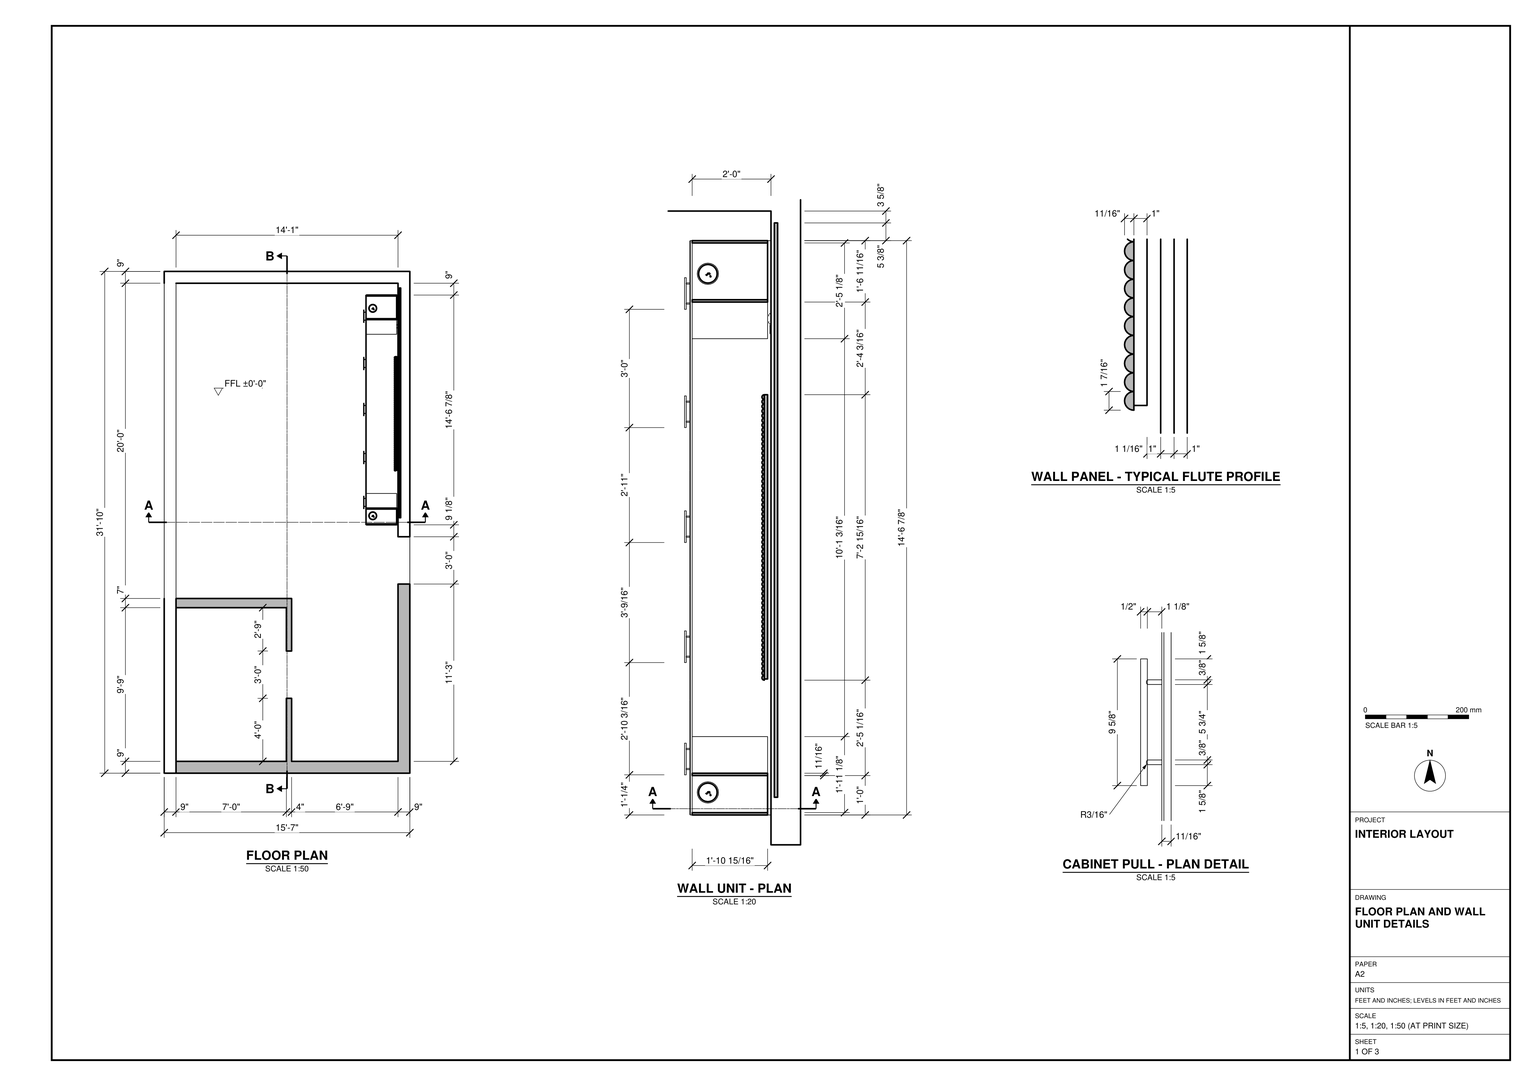
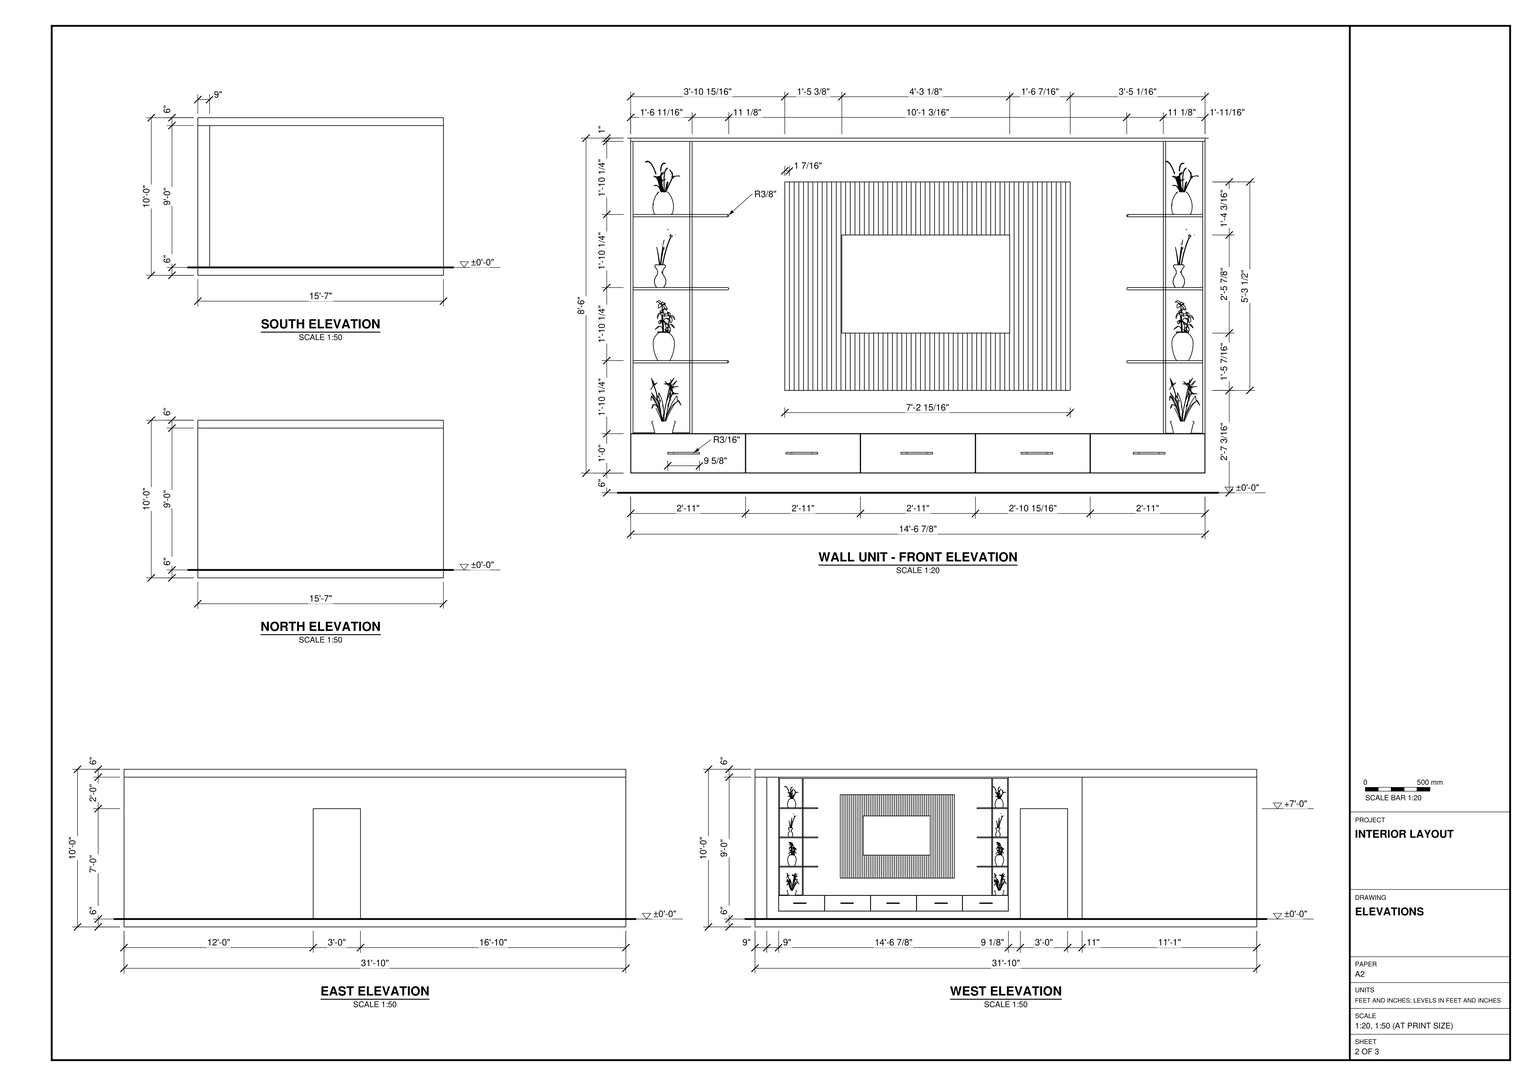
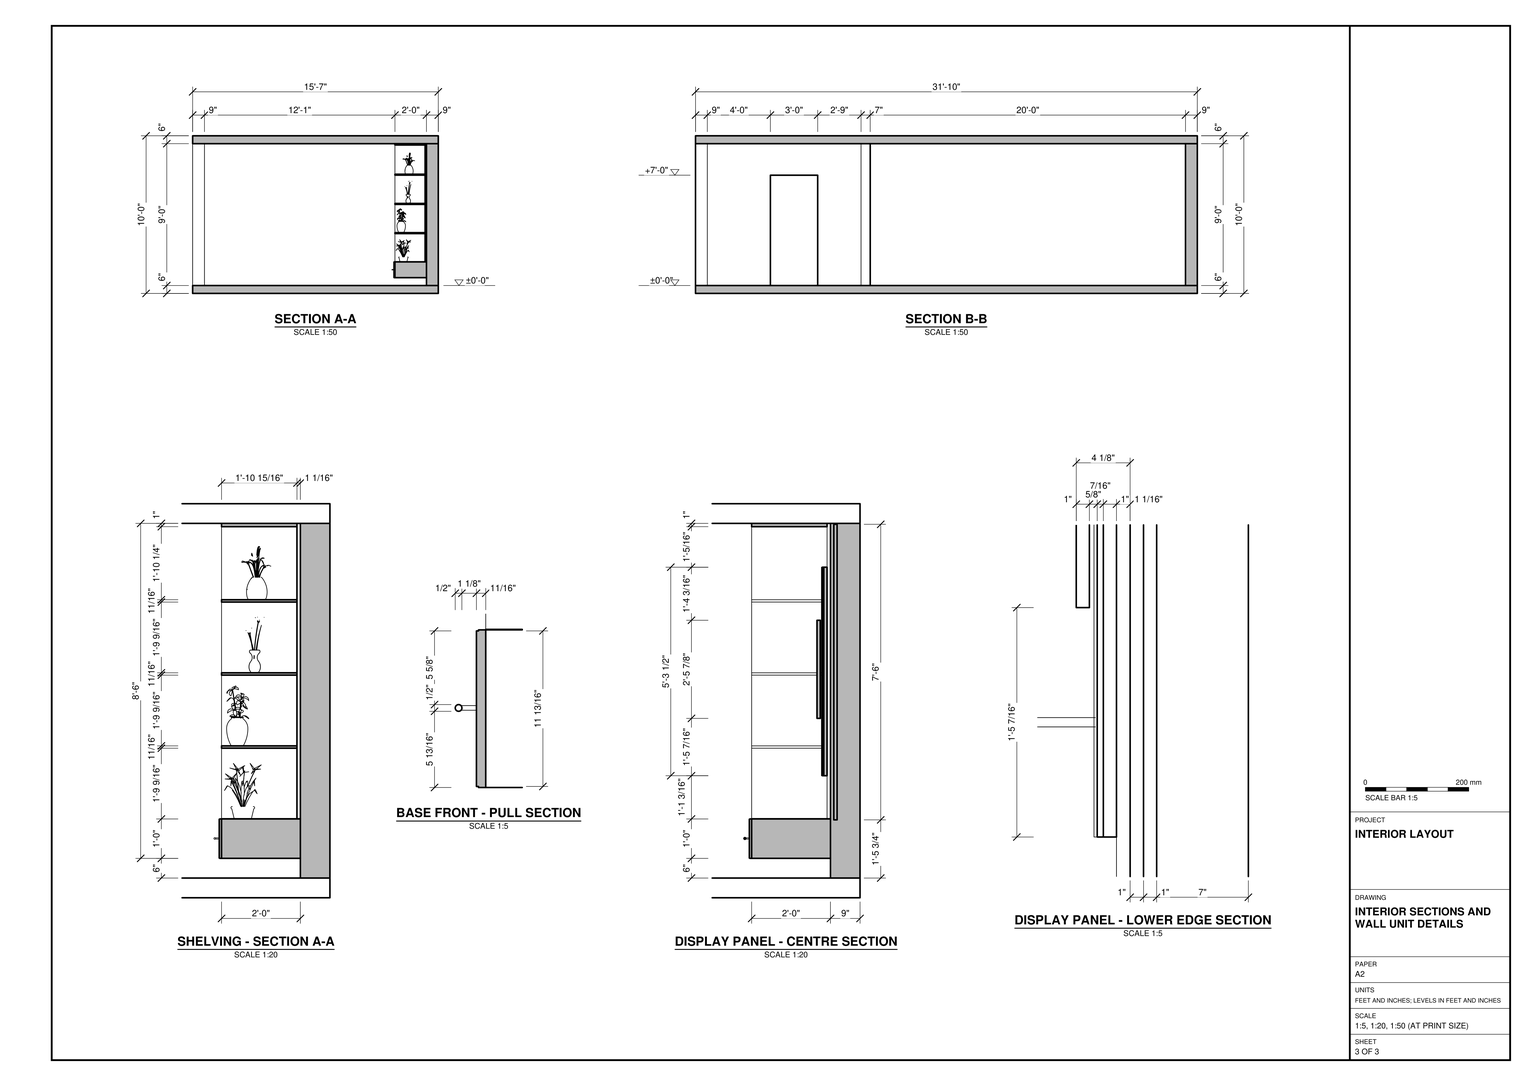
Build the interior in SketchUp from task_files/diagram_01.pdf. Work in feet and inches. The shell is 15'-7" wide, 31'-10" long and 10'-0" high, with one finished floor at ±0'-0". Use the floor plan to locate the walls and the sections to set the 6" floor and roof slabs around the 9'-0" clear interior height. Follow the wall thicknesses shown: 9" at the perimeter, 7" at the cross partition and 4" at the side partition of the small southwest room. Leave the doorway openings in the positions drawn.

Fit the display unit against the east wall, between the north end of the main space and the east doorway. Use the joinery plan, front elevation and sections together to set its length, depth and clearance above the floor. Divide the floating base into five fronts with horizontal pulls. Build the open shelves at both ends, the continuous top and the vertically fluted central panel with its smaller rectangular display face. Model the panel relief and the projection of the pulls as shown in the details. Shelf plants, vases and other loose decor may be any suitable library components placed as shown.

Keep the walls, floor slab and roof slab as separate shell groups or components, and group each furniture or joinery piece separately. Use components for repeated parts. Save one SketchUp model as output_files/single_storey_interior_with_a_built_in_display_wall.skp.

# SketchUp Ruby script. Lengths in inches.
U = 1.inch
M = Sketchup.active_model
def pt(a) = Geom::Point3d.new(a.map { |v| v * U })
def face(e, loops, mat)
  f = e.add_face(loops[0].map { |a| pt(a) })
  loops[1..].each { |l| e.add_face(l.map { |a| pt(a) }).erase! }
  f.material = f.back_material = mat if mat
  f
end
# faces: each face lists its corners as indices into pts; further lists are holes
def faces(e, pts, list, mat = nil) = list.each { |f| face(e, (f[0].is_a?(Array) ? f : [f]).map { |l| l.map { |i| pts[i] } }, mat) }
# xy, xz, yz: faces in a plane at the given z, y or x. An outline is a flat list of corners, or four numbers for a rectangle; further outlines are holes
def ring(l) = l.size == 4 ? [[l[0], l[1]], [l[2], l[1]], [l[2], l[3]], [l[0], l[3]]] : l.each_slice(2).to_a
def flat(e, list, mat, &to3) = list.each { |f| face(e, (f[0].is_a?(Array) ? f : [f]).map { |l| ring(l).map { |u, v| to3.(u, v) } }, mat) }
def xy(e, z, list, mat = nil) = flat(e, list, mat) { |x, y| [x, y, z] }
def xz(e, y, list, mat = nil) = flat(e, list, mat) { |x, z| [x, y, z] }
def yz(e, x, list, mat = nil) = flat(e, list, mat) { |y, z| [x, y, z] }
def lines(e, pts, list) = list.each { |a, b| e.add_line(pt(pts[a]), pt(pts[b])) }
# prism: a flat outline (further loops are holes) pulled along v
def prism(e, loops, v, mat = nil)
  f = face(e, loops, mat); d = Geom::Vector3d.new(v.map { |x| x * U })
  f.pushpull(f.normal.samedirection?(d) ? d.length : -d.length)
end
def box(e, o, s, mat = nil) = prism(e, [[o, [o[0] + s[0], o[1], o[2]], [o[0] + s[0], o[1] + s[1], o[2]], [o[0], o[1] + s[1], o[2]]]], [0, 0, s[2]], mat)
def at(x, y, z, deg = 0) = Geom::Transformation.translation(pt([x, y, z])) * Geom::Transformation.rotation(ORIGIN, Z_AXIS, deg.degrees)
def axes(o, x, y, z) = Geom::Transformation.new([*x, 0, *y, 0, *z, 0, *pt(o).to_a, 1])
def part(name) = M.definitions.add(name)
# library, detail: a bought-in or finely detailed component or shape, given as its bounding box
def library(name, o, s) = part(name).tap { |d| box(d.entities, o, s) }
def detail(e, o, s) = box(e.add_group.entities, o, s)
def put(e, d, t, mat = nil) = e.add_instance(d, t).tap { |i| i.material = mat if mat }
def group(e, t, mat = nil) = e.add_group.tap { |g| g.transformation = t; g.material = mat if mat }.entities
root = M.entities
M.materials.add("CLC2-HANDLES-BT - LANSA").color = [177, 177, 177]
M.materials.add("CLC2-PC-Blanc INTER").color = [249, 249, 249]
M.materials.add("[Color M00]").color = [255, 255, 255]
M.materials.add("[Color M04]").color = [142, 142, 142]
M.materials.add("[Color M09]").color = [0, 0, 0]
M.materials.add("[Wood Cherry Original]").color = [152, 86, 42]
M.materials.add("[Wood Lumber ButtJoined]").color = [198, 184, 135]
c1 = library("7-VASEFLEURS CLC2",[-5.69,-5.69,0],[10.79,12.36,17.9])
c2 = library("3-VASEFLEURS CLC2",[-4.45,-7.875,0],[9.14,10,23.05])
c3 = library("1-VASEFLEURS CLC2",[-4.93,-4.36,0],[9.88,8.02,19.93])
c4 = library("5-VASEFLEURS CLC2",[-6.43,-5.48,0.34],[13.26,9.94,17.7])
c5 = library("3-PRISEELC CLC2",[-1.57,-1.57,0],[3.14,3.14,0.6875])
c6 = part("CLC2-Ele02")
prism(c6.entities,[[[0.84,-0.32,0.16],[0.84,-0.33,0.02],[0.84,-0.34,-0.125],[0.84,-0.36,-0.27],[0.84,-0.39,-0.41],[0.84,-0.43,-0.55],[0.84,-0.47,-0.68],[0.84,-0.51,-0.82],[0.84,-0.2,-0.84],[0.84,-0.07,0.84],[0.84,-0.375,0.87],[0.84,-0.35,0.73],[0.84,-0.33,0.59],[0.84,-0.32,0.44],[0.84,-0.32,0.3]]],[-0.83,0,0],"CLC2-PC-Blanc INTER")
prism(c6.entities,[[[-0.01,-0.32,0.16],[-0.01,-0.33,0.02],[-0.01,-0.34,-0.125],[-0.01,-0.36,-0.27],[-0.01,-0.39,-0.41],[-0.01,-0.43,-0.55],[-0.01,-0.47,-0.68],[-0.01,-0.51,-0.82],[-0.01,-0.2,-0.84],[-0.01,-0.07,0.84],[-0.01,-0.375,0.87],[-0.01,-0.35,0.73],[-0.01,-0.33,0.59],[-0.01,-0.32,0.44],[-0.01,-0.32,0.3]]],[-0.83,0,0],"CLC2-PC-Blanc INTER")
xy(c6.entities,-1.57,[[-1.44,-0.19,1.44,0]],"CLC2-PC-Blanc INTER")
xy(c6.entities,-1.5,[[-1.375,-0.12,1.375,0]],"CLC2-PC-Blanc INTER")
xy(c6.entities,-0.87,[[-0.85,-0.29,0.85,-0.12]],"CLC2-PC-Blanc INTER")
xy(c6.entities,0.87,[[-0.85,-0.29,0.85,-0.12]],"CLC2-PC-Blanc INTER")
xy(c6.entities,1.5,[[-1.375,-0.12,1.375,0]],"CLC2-PC-Blanc INTER")
xy(c6.entities,1.57,[[-1.44,-0.19,1.44,0]],"CLC2-PC-Blanc INTER")
xz(c6.entities,-0.12,[[[-1.375,-1.5,-1.41,-1.3,-1.4375,-1.04,-1.46,-0.78,-1.48,-0.52,-1.5,0,-1.48,0.52,-1.46,0.78,-1.4375,1.04,-1.41,1.3,-1.375,1.5,1.375,1.5,1.41,1.3,1.4375,1.04,1.46,0.78,1.48,0.52,1.5,0,1.48,-0.52,1.46,-0.78,1.4375,-1.04,1.41,-1.3,1.375,-1.5],[-0.85,-0.87,0.85,0.87]]],"CLC2-PC-Blanc INTER")
xz(c6.entities,0,[[-1.44,-1.57,-1.48,-1.3125,-1.51,-1.05,-1.54,-0.79,-1.56,-0.53,-1.57,-0.26,-1.57,0.26,-1.56,0.53,-1.54,0.79,-1.51,1.05,-1.48,1.3125,-1.44,1.57,0,1.57,0,1.5,-1.375,1.5,-1.41,1.3,-1.4375,1.04,-1.46,0.78,-1.48,0.52,-1.5,0,-1.48,-0.52,-1.46,-0.78,-1.4375,-1.04,-1.41,-1.3,-1.375,-1.5,0,-1.5,0,-1.57],[0,-1.57,0,-1.5,1.375,-1.5,1.41,-1.3,1.4375,-1.04,1.46,-0.78,1.48,-0.52,1.5,0,1.48,0.52,1.46,0.78,1.4375,1.04,1.41,1.3,1.375,1.5,0,1.5,0,1.57,1.44,1.57,1.48,1.3125,1.51,1.05,1.54,0.79,1.56,0.53,1.57,0.26,1.57,-0.26,1.56,-0.53,1.54,-0.79,1.51,-1.05,1.48,-1.3125,1.44,-1.57]],"CLC2-PC-Blanc INTER")
yz(c6.entities,-1.57,[[-0.0625,-0.26,-0.06,0,0,0,0,-0.26],[-0.06,0,-0.0625,0.26,0,0.26,0,0]],"CLC2-PC-Blanc INTER")
yz(c6.entities,-0.85,[[-0.29,-0.87,-0.12,-0.87,-0.12,0.87,-0.29,0.87,-0.29,0.79,-0.3125,0.53,-0.32,0.26,-0.33,0,-0.32,-0.26,-0.3125,-0.53,-0.29,-0.79]],"CLC2-PC-Blanc INTER")
yz(c6.entities,0.85,[[-0.29,-0.87,-0.29,-0.79,-0.3125,-0.53,-0.32,-0.26,-0.33,0,-0.32,0.26,-0.3125,0.53,-0.29,0.79,-0.29,0.87,-0.12,0.87,-0.12,-0.87]],"CLC2-PC-Blanc INTER")
yz(c6.entities,1.57,[[-0.0625,-0.26,0,-0.26,0,0,-0.06,0],[-0.06,0,0,0,0,0.26,-0.0625,0.26]],"CLC2-PC-Blanc INTER")
p = [[-1.32,-0.3125,0.53],[-1.34,-0.29,0.79],[-1.37,-0.27,1.05],[-1.4,-0.23,1.3125],[-1.44,-0.19,1.57],[-1.48,-0.15,1.3125],
  [-1.51,-0.12,1.05],[-1.54,-0.09,0.79],[-1.56,-0.07,0.53],[-1.57,-0.0625,0.26],[-1.57,-0.06,0],[-1.57,-0.0625,-0.26],
  [-1.56,-0.07,-0.53],[-1.54,-0.09,-0.79],[-1.51,-0.12,-1.05],[-1.48,-0.15,-1.3125],[-1.44,-0.19,-1.57],[-1.4,-0.23,-1.3125],
  [-1.37,-0.27,-1.05],[-1.34,-0.29,-0.79],[-1.32,-0.3125,-0.53],[-1.31,-0.32,-0.26],[-1.3,-0.33,0],[-1.31,-0.32,0.26],
  [1.34,-0.29,0.79],[1.32,-0.3125,0.53],[1.31,-0.32,0.26],[1.3,-0.33,0],[1.31,-0.32,-0.26],[1.32,-0.3125,-0.53],
  [1.34,-0.29,-0.79],[1.37,-0.27,-1.05],[1.4,-0.23,-1.3125],[1.44,-0.19,-1.57],[1.48,-0.15,-1.3125],[1.51,-0.12,-1.05],
  [1.54,-0.09,-0.79],[1.56,-0.07,-0.53],[1.57,-0.0625,-0.26],[1.57,-0.06,0],[1.57,-0.0625,0.26],[1.56,-0.07,0.53],
  [1.54,-0.09,0.79],[1.51,-0.12,1.05],[1.48,-0.15,1.3125],[1.44,-0.19,1.57],[1.4,-0.23,1.3125],[1.37,-0.27,1.05],
  [-1.44,0,-1.57],[-1.48,0,-1.3125],[1.44,0,-1.57],[1.48,0,-1.3125],[-1.375,0,-1.5],[-1.41,0,-1.3],
  [-1.41,-0.12,-1.3],[-1.375,-0.12,-1.5],[1.41,0,-1.3],[1.375,0,-1.5],[1.375,-0.12,-1.5],[1.41,-0.12,-1.3],
  [-1.51,0,-1.05],[1.51,0,-1.05],[-1.4375,0,-1.04],[-1.4375,-0.12,-1.04],[1.4375,0,-1.04],[1.4375,-0.12,-1.04],
  [0.85,-0.29,-0.87],[-0.85,-0.29,-0.87],[-0.85,-0.29,-0.79],[-1.33,-0.29,-0.79],[1.33,-0.29,-0.79],[0.85,-0.29,-0.79],
  [-1.54,0,-0.79],[1.54,0,-0.79],[-1.46,0,-0.78],[-1.46,-0.12,-0.78],[1.46,0,-0.78],[1.46,-0.12,-0.78],
  [-0.85,-0.3125,-0.53],[0.85,-0.3125,-0.53],[-1.56,0,-0.53],[-1.48,0,-0.52],[-1.48,-0.12,-0.52],[1.48,0,-0.52],
  [1.48,-0.12,-0.52],[1.56,0,-0.53],[-0.85,-0.32,-0.26],[0.85,-0.32,-0.26],[-1.57,0,-0.26],[-1.49,0,-0.26],
  [-1.49,-0.12,-0.26],[1.49,0,-0.26],[1.49,-0.12,-0.26],[1.57,0,-0.26],[-0.85,-0.33,0],[0.85,-0.33,0],
  [-1.5,0,0],[-1.5,-0.12,0],[1.5,0,0],[1.5,-0.12,0],[-0.85,-0.32,0.26],[0.85,-0.32,0.26],
  [-1.49,0,0.26],[-1.49,-0.12,0.26],[1.49,0,0.26],[1.49,-0.12,0.26],[-0.85,-0.3125,0.53],[0.85,-0.3125,0.53],
  [-1.57,0,0.26],[-1.56,0,0.53],[-1.48,0,0.52],[-1.48,-0.12,0.52],[1.48,0,0.52],[1.48,-0.12,0.52],
  [1.57,0,0.26],[1.56,0,0.53],[-0.85,-0.29,0.79],[-1.33,-0.29,0.79],[1.33,-0.29,0.79],[0.85,-0.29,0.79],
  [-1.54,0,0.79],[-1.46,0,0.78],[-1.46,-0.12,0.78],[1.46,0,0.78],[1.46,-0.12,0.78],[1.54,0,0.79],
  [-0.85,-0.29,0.87],[0.85,-0.29,0.87],[-1.4375,0,1.04],[-1.4375,-0.12,1.04],[-1.51,0,1.05],[1.4375,0,1.04],
  [1.4375,-0.12,1.04],[1.51,0,1.05],[-1.41,0,1.3],[-1.41,-0.12,1.3],[1.41,0,1.3],[1.41,-0.12,1.3],
  [-1.48,0,1.3125],[1.48,0,1.3125],[-1.44,0,1.57],[1.44,0,1.57],[-1.375,0,1.5],[-1.375,-0.12,1.5],
  [1.375,0,1.5],[1.375,-0.12,1.5]]
faces(c6.entities,p,[[0,1,2,3,4,5,6,7,8,9,10,11,12,13,14,15,16,17,18,19,20,21,22,23],[24,25,26,27,28,29,30,31,32,33,34,35,36,37,38,39,40,41,42,43,44,45,46,47],[48,16,15,49],[33,50,51,34],[52,53,54,55],[56,57,58,59],[49,15,14,60],[34,51,61,35],
  [53,62,63,54],[64,56,59,65],[60,14,13,72],[35,61,73,36],[62,74,75,63],[76,64,65,77],[72,13,12,80],[74,81,82,75],
  [83,76,77,84],[36,73,85,37],[80,12,11,88],[81,89,90,82],[91,83,84,92],[37,85,93,38],[89,96,97,90],[98,91,92,99],
  [96,102,103,97],[104,98,99,105],[108,9,8,109],[102,110,111,103],[112,104,105,113],[40,114,115,41],[109,8,7,120],[110,121,122,111],
  [123,112,113,124],[41,115,125,42],[121,128,129,122],[120,7,6,130],[131,123,124,132],[42,125,133,43],[128,134,135,129],[136,131,132,137],
  [130,6,5,138],[43,133,139,44],[138,5,4,140],[44,139,141,45],[134,142,143,135],[144,136,137,145]],"CLC2-PC-Blanc INTER")
faces(c6.entities,p,[[32,17,16,33],[31,18,17,32],[66,67,68,69,19,18,31,30,70,71],[69,68,78,20,19],[71,70,30,29,79],[20,78,86,21],[79,29,28,87],[21,86,94,22],
  [87,28,27,95],[22,94,100,23],[95,27,26,101],[23,100,106,0],[101,26,25,107],[0,106,116,117,1],[107,25,24,118,119],[116,126,127,119,118,24,47,2,1,117],
  [46,3,2,47],[4,3,46,45]],"[Color M04]")
c7 = part("2-PRISEELC CLC2")
put(c7.entities,c6,axes([0,0,0],[1,0,0],[0,0,-1],[0,1,0]))
c8 = part("3-POIGNEE CLC2")
yz(c8.entities,-4.823,[[0,1.102,-0.066,1.111,-0.128,1.137,-0.181,1.177,-0.222,1.23,-0.247,1.292,-0.256,1.358,-0.247,1.425,-0.222,1.486,-0.181,1.539,-0.128,1.58,-0.066,1.605,0,1.614,0.066,1.605,0.128,1.58,0.181,1.539,0.222,1.486,0.247,1.425,0.256,1.358,0.247,1.292,0.222,1.23,0.181,1.177,0.128,1.137,0.066,1.111]],"CLC2-HANDLES-BT - LANSA")
yz(c8.entities,4.823,[[0,1.102,0.066,1.111,0.128,1.137,0.181,1.177,0.222,1.23,0.247,1.292,0.256,1.358,0.247,1.425,0.222,1.486,0.181,1.539,0.128,1.58,0.066,1.605,0,1.614,-0.066,1.605,-0.128,1.58,-0.181,1.539,-0.222,1.486,-0.247,1.425,-0.256,1.358,-0.247,1.292,-0.222,1.23,-0.181,1.177,-0.128,1.137,-0.066,1.111]],"CLC2-HANDLES-BT - LANSA")
p = [[-3.135,-0.156,0],[-3.135,-0.156,1.159],[-3.173,-0.129,1.138],[-3.173,-0.128,1.137],[-3.173,-0.129,0],[-3.092,-0.172,0],
  [-3.092,-0.172,1.171],[-3.046,-0.177,1.175],[-3.056,-0.176,0],[-3.046,-0.177,0],[-2.922,-0.122,0],[-2.922,-0.122,1.134],
  [-2.929,-0.127,1.137],[-2.958,-0.151,1.155],[-2.958,-0.151,0],[-3,-0.17,0],[-3,-0.17,1.169],[2.967,-0.156,0],
  [2.967,-0.156,1.159],[2.93,-0.129,1.138],[2.93,-0.129,0],[3.056,-0.177,1.175],[3.01,-0.172,1.171],[3.01,-0.172,0],
  [3.046,-0.176,0],[3.056,-0.177,0],[3.18,-0.122,0],[3.18,-0.122,1.134],[3.173,-0.127,1.137],[3.144,-0.151,1.155],
  [3.144,-0.151,0],[3.102,-0.17,1.169],[3.102,-0.17,0],[-3.174,-0.128,1.137],[-3.202,-0.093,1.122],[-3.202,-0.093,0],
  [-3.221,-0.051,0],[-3.221,-0.051,1.109],[-3.228,-0.005,1.103],[-3.228,-0.005,0],[-3.214,-0.066,1.111],[-2.895,-0.084,0],
  [-2.895,-0.084,1.119],[-2.879,-0.041,0],[-2.879,-0.041,1.108],[-2.888,-0.066,1.111],[2.881,-0.051,0],[2.881,-0.051,1.109],
  [2.874,-0.005,1.103],[2.874,-0.005,0],[2.929,-0.128,1.137],[2.9,-0.093,1.122],[2.9,-0.093,0],[2.888,-0.066,1.111],
  [3.224,-0.041,0],[3.224,-0.041,1.108],[3.214,-0.066,1.111],[3.207,-0.084,1.119],[3.207,-0.084,0],[-3.224,0.041,0],
  [-3.224,0.041,1.108],[-3.214,0.067,1.111],[-3.207,0.084,1.118],[-3.207,0.084,0],[-3.228,0.001,1.102],[-2.874,0.005,0],
  [-2.874,0.005,1.103],[-2.875,0.001,1.102],[-2.881,0.051,0],[-2.881,0.051,1.109],[2.875,0.001,1.102],[2.879,0.041,1.108],
  [2.879,0.041,0],[2.889,0.067,1.111],[2.895,0.084,1.118],[2.895,0.084,0],[3.228,0.005,0],[3.228,0.005,1.103],
  [3.228,0.001,1.102],[3.221,0.051,0],[3.221,0.051,1.109],[-3.18,0.122,0],[-3.18,0.122,1.134],[-3.172,0.128,1.137],
  [-3.144,0.151,1.154],[-3.144,0.151,0],[-2.967,0.156,0],[-2.967,0.156,1.158],[-2.93,0.129,1.137],[-2.93,0.129,0],
  [-2.929,0.128,1.137],[-2.9,0.093,1.122],[-2.9,0.093,0],[-2.889,0.067,1.111],[2.922,0.122,1.134],[2.922,0.122,0],
  [2.931,0.128,1.137],[2.958,0.151,1.154],[2.958,0.151,0],[3.135,0.156,0],[3.135,0.156,1.158],[3.173,0.129,1.137],
  [3.173,0.129,0],[3.202,0.093,0],[3.202,0.093,1.122],[3.214,0.067,1.111],[3.173,0.128,1.137],[-3.102,0.17,1.168],
  [-3.102,0.17,0],[-3.056,0.177,0],[-3.056,0.177,1.174],[-3.01,0.172,1.17],[-3.01,0.172,0],[3,0.17,1.168],
  [3,0.17,0],[3.046,0.177,1.174],[3.046,0.177,0],[3.092,0.172,1.17],[3.092,0.172,0],[-4.823,-0.128,1.137],
  [4.823,-0.128,1.137],[4.823,-0.181,1.177],[-4.823,-0.181,1.177],[-4.823,-0.066,1.111],[4.823,-0.066,1.111],[-4.823,0,1.102],
  [4.823,0,1.102],[-4.823,0.066,1.111],[4.823,0.066,1.111],[4.823,0.181,1.177],[4.823,0.128,1.137],[3.516,0.128,1.137],
  [-4.823,0.128,1.137],[-4.823,0.181,1.177],[-4.823,-0.247,1.292],[-4.823,-0.222,1.23],[4.823,-0.222,1.23],[4.823,-0.247,1.292],
  [-4.823,0.222,1.23],[-4.823,0.247,1.292],[4.823,0.247,1.292],[4.823,0.222,1.23],[-4.823,-0.256,1.358],[4.823,-0.256,1.358],
  [-4.823,0.256,1.358],[4.823,0.256,1.358],[-4.823,-0.247,1.425],[4.823,-0.247,1.425],[-4.823,-0.222,1.486],[4.823,-0.222,1.486],
  [-4.823,0.247,1.425],[4.823,0.247,1.425],[-4.823,0.222,1.486],[4.823,0.222,1.486],[-4.823,-0.128,1.58],[-4.823,-0.181,1.539],
  [4.823,-0.181,1.539],[4.823,-0.128,1.58],[-4.823,0.181,1.539],[-4.823,0.128,1.58],[4.823,0.128,1.58],[4.823,0.181,1.539],
  [-4.823,0,1.614],[-4.823,-0.066,1.605],[4.823,-0.066,1.605],[4.823,0,1.614],[-4.823,0.066,1.605],[4.823,0.066,1.605]]
faces(c8.entities,p,[[0,1,2,3,4],[5,6,1,0],[7,6,5,8,9],[10,11,12,13,14],[15,16,7,9],[14,13,16,15],[17,18,19,20],[21,22,23,24,25],
  [23,22,18,17],[26,27,28,29,30],[30,29,31,32],[32,31,21,25],[4,3,2,33,34,35],[36,37,38,39],[35,34,40,37,36],[41,42,11,10],
  [43,44,45,42,41],[46,47,48,49],[20,19,50,51,52],[52,51,53,47,46],[54,55,56,57,58],[58,57,27,26],[59,60,61,62,63],[39,38,64,60,59],
  [65,66,67,44,43],[68,69,66,65],[49,48,70,71,72],[72,71,73,74,75],[76,77,78,55,54],[79,80,77,76],[81,82,83,84,85],[63,62,82,81],
  [86,87,88,89],[89,88,90,91,92],[92,91,93,69,68],[75,74,94,95],[95,94,96,97,98],[99,100,101,102],[103,104,105,80,79],[102,101,106,104,103],
  [85,84,107,108],[109,110,111,112],[108,107,110,109],[112,111,87,86],[98,97,113,114],[114,113,115,116],[116,115,117,118],[118,117,100,99],
  [119,33,12,50,28,120,121,122],[123,40,45,53,56,124,120,28,50,12,33,119],[125,64,38,37,40,123],[64,67,44,45,40,37,38],[67,70,48,47,53,45,44],[70,78,55,56,53,47,48],[124,56,55,78,126],[127,61,60,64,125],
  [61,93,69,66,67,64,60],[93,73,71,70,67,66,69],[78,70,71,73,105,80,77],[126,78,77,80,105,128],[129,130,131,101,96,88,83,132,133],[131,130,128,105,73,93,61,127,132,83,88,96,101],[134,135,136,137],[135,122,121,136],
  [138,139,140,141],[133,138,141,129],[142,134,137,143],[139,144,145,140],[146,142,143,147],[148,146,147,149],[144,150,151,145],[150,152,153,151],
  [154,155,156,157],[155,148,149,156],[158,159,160,161],[152,158,161,153],[162,163,164,165],[163,154,157,164],[166,162,165,167],[159,166,167,160]],"CLC2-HANDLES-BT - LANSA")
c9 = part("Group22\#2")
xy(c9.entities,0,[[1172.2,321,1172.2,703,1359.2,703,1359.2,501,1350.2,501,1350.2,694,1181.2,694,1181.2,321],[1181.2,321,1181.2,330,1265.2,330,1265.2,378,1269.2,378,1269.2,330,1350.2,330,1350.2,465,1359.2,465,1359.2,321],[1265.2,414,1265.2,447,1181.2,447,1181.2,454,1269.2,454,1269.2,414]])
xy(c9.entities,84,[[1265.2,378,1269.2,414],[1350.2,465,1359.2,501]])
xy(c9.entities,108,[[1172.2,321,1181.2,454],[1181.2,321,1359.2,321,1359.2,703,1172.2,703,1172.2,694,1350.2,694,1350.2,330,1269.2,330,1269.2,454,1181.2,454,1181.2,447,1265.2,447,1265.2,330,1181.2,330],[1172.2,454,1181.2,694]])
xz(c9.entities,321,[[1181.2,0,1359.2,108]])
xz(c9.entities,321,[[1172.2,0,1181.2,108]],"[Color M00]")
xz(c9.entities,330,[[1181.2,0,1265.2,108],[1269.2,0,1350.2,108]])
xz(c9.entities,378,[[1265.2,0,1269.2,84]])
xz(c9.entities,414,[[1265.2,0,1269.2,84]])
xz(c9.entities,447,[[1181.2,0,1265.2,108]])
xz(c9.entities,454,[[1181.2,0,1269.2,108]])
xz(c9.entities,465,[[1350.2,0,1359.2,84]])
xz(c9.entities,501,[[1350.2,0,1359.2,84]])
xz(c9.entities,694,[[1181.2,0,1350.2,108]],"[Color M00]")
xz(c9.entities,703,[[1172.2,0,1359.2,108]])
yz(c9.entities,1172.2,[[321,0,454,108],[694,0,703,108]],"[Color M00]")
yz(c9.entities,1181.2,[[321,0,330,108],[447,0,454,108]])
yz(c9.entities,1181.2,[[330,0,447,108]],"[Color M00]")
yz(c9.entities,1265.2,[[330,0,330,108,447,108,447,0,414,0,414,84,378,84,378,0]])
yz(c9.entities,1269.2,[[330,0,378,0,378,84,414,84,414,0,454,0,454,108,330,108]])
yz(c9.entities,1350.2,[[330,0,330,108,694,108,694,0,501,0,501,84,465,84,465,0]],"[Wood Lumber ButtJoined]")
yz(c9.entities,1359.2,[[321,0,465,0,465,84,501,84,501,0,703,0,703,108,321,108]])
c10 = part("Group\#7")
box(c10.entities,[-22.96,0,0],[22.96,0.71,89])
c11 = part("Vertical slat")
prism(c11.entities,[[[0.375,0.75,-33.42],[0.375,0,-33.42],[0.28,0.01,-33.42],[0.1875,0.05,-33.42],[0.11,0.11,-33.42],[0.05,0.1875,-33.42],[0.01,0.28,-33.42],[0,0.375,-33.42],[0.01,0.47,-33.42],[0.05,0.5625,-33.42],[0.11,0.64,-33.42],[0.1875,0.7,-33.42],[0.28,0.74,-33.42]]],[0,0,33.42],"[Wood Cherry Original]")
xy(root,18,[[154,189.1,178,364]])
xy(root,18.04,[[154,189.1,178,364]],"[Wood Lumber ButtJoined]")
xz(root,189.1,[[154,18,178,18.04]])
xz(root,364,[[154,18,178,18.04]])
yz(root,154,[[189.1,18,364,18.04]])
yz(root,176.96,[[189.81,18.14,201.1,39.54],[346,18.28,363.29,39.54],[189.81,40.25,201.1,61.79],[346,40.25,363.29,61.79],[189.81,62.5,201.1,84.04],
  [346,62.5,363.29,84.04],[189.81,84.75,201.1,107],[346,84.75,363.29,107]],"[Wood Lumber ButtJoined]")
yz(root,178,[[189.1,18,364,18.04]])
put(root,c1,at(164.72,354.04,84.47))
put(root,c2,axes([164.11,355.05,62.22],[0.82,0,0],[0,0.82,0],[0,0,0.82]))
put(root,c3,at(158.79,353.86,39.97))
put(root,c4,at(160.43,353.92,17.66))
put(root,c1,at(164.72,196.1,84.47))
put(root,c3,at(158.79,195.92,39.97))
put(root,c2,axes([164.11,197.11,62.22],[0.82,0,0],[0,0.82,0],[0,0,0.82]))
put(root,c4,at(160.43,195.98,17.66))
put(root,c5,axes([178,340.19,29.48],[0,-1,0],[0,0,1],[-1,0,0]))
put(root,c7,axes([178,336.94,29.48],[0,-1,0],[0,0,1],[-1,0,0]))
put(root,c8,axes([153.29,276.89,12.06],[0,-1,0],[0,0,1],[-1,0,0]))
put(root,c8,axes([153.29,240.33,12.06],[0,-1,0],[0,0,1],[-1,0,0]))
put(root,c8,axes([153.29,206.14,12.06],[0,-1,0],[0,0,1],[-1,0,0]))
put(root,c8,axes([153.29,311.89,12.06],[0,-1,0],[0,0,1],[-1,0,0]))
put(root,c8,axes([153.29,347.89,12.06],[0,-1,0],[0,0,1],[-1,0,0]))
put(root,c9,at(-1172.2,-321,0))
g1 = group(root,at(154,189.1,6))
box(g1,[0,0,0],[24,174.9,12])
g2 = group(root,at(179.02,194.49,17.72))
box(g2,[0,0,0],[1,174.9,90])
g3 = group(root,at(176.96,363.29,18),"[Wood Lumber ButtJoined]")
box(g3,[-22.96,0,0],[22.96,0.71,89])
put(root,c10,at(176.96,189.1,18),"[Wood Lumber ButtJoined]")
g4 = group(root,at(176.96,189.1,107))
box(g4,[-22.96,0,0],[22.96,174.9,1],"[Wood Cherry Original]")
put(root,c10,at(176.96,345.29,18),"[Wood Lumber ButtJoined]")
put(root,c10,at(176.96,201.1,18),"[Wood Lumber ButtJoined]")
g5 = group(root,at(176.96,230.51,31.16))
xy(g5,0,[[-1,0,0,86.5625]])
xy(g5,63.5,[[-1,0,0,86.5625]])
xz(g5,0,[[-1,0,0,63.5]])
xz(g5,86.5625,[[-1,0,0,63.5]])
yz(g5,-1,[[0,0,86.5625,63.5]])
yz(g5,0,[[0,0,86.5625,63.5]])
put(g5,c11,axes([-1.71,85.14,63.5],[1.9,0,0],[0,1.9,0],[0,0,1.9]))
put(g5,c11,axes([-1.71,83.71,63.5],[1.9,0,0],[0,1.9,0],[0,0,1.9]))
put(g5,c11,axes([-1.71,82.29,63.5],[1.9,0,0],[0,1.9,0],[0,0,1.9]))
put(g5,c11,axes([-1.71,80.86,63.5],[1.9,0,0],[0,1.9,0],[0,0,1.9]))
put(g5,c11,axes([-1.71,79.4375,63.5],[1.9,0,0],[0,1.9,0],[0,0,1.9]))
put(g5,c11,axes([-1.71,78.01,63.5],[1.9,0,0],[0,1.9,0],[0,0,1.9]))
put(g5,c11,axes([-1.71,76.59,63.5],[1.9,0,0],[0,1.9,0],[0,0,1.9]))
put(g5,c11,axes([-1.71,75.16,63.5],[1.9,0,0],[0,1.9,0],[0,0,1.9]))
put(g5,c11,axes([-1.71,73.74,63.5],[1.9,0,0],[0,1.9,0],[0,0,1.9]))
put(g5,c11,axes([-1.71,72.3125,63.5],[1.9,0,0],[0,1.9,0],[0,0,1.9]))
put(g5,c11,axes([-1.71,70.89,63.5],[1.9,0,0],[0,1.9,0],[0,0,1.9]))
put(g5,c11,axes([-1.71,69.46,63.5],[1.9,0,0],[0,1.9,0],[0,0,1.9]))
put(g5,c11,axes([-1.71,68.04,63.5],[1.9,0,0],[0,1.9,0],[0,0,1.9]))
put(g5,c11,axes([-1.71,66.61,63.5],[1.9,0,0],[0,1.9,0],[0,0,1.9]))
put(g5,c11,axes([-1.71,65.1875,63.5],[1.9,0,0],[0,1.9,0],[0,0,1.9]))
put(g5,c11,axes([-1.71,63.76,63.5],[1.9,0,0],[0,1.9,0],[0,0,1.9]))
put(g5,c11,axes([-1.71,62.34,63.5],[1.9,0,0],[0,1.9,0],[0,0,1.9]))
put(g5,c11,axes([-1.71,60.91,63.5],[1.9,0,0],[0,1.9,0],[0,0,1.9]))
put(g5,c11,axes([-1.71,59.49,63.5],[1.9,0,0],[0,1.9,0],[0,0,1.9]))
put(g5,c11,axes([-1.71,58.0625,63.5],[1.9,0,0],[0,1.9,0],[0,0,1.9]))
put(g5,c11,axes([-1.71,56.64,63.5],[1.9,0,0],[0,1.9,0],[0,0,1.9]))
put(g5,c11,axes([-1.71,55.21,63.5],[1.9,0,0],[0,1.9,0],[0,0,1.9]))
put(g5,c11,axes([-1.71,53.79,63.5],[1.9,0,0],[0,1.9,0],[0,0,1.9]))
put(g5,c11,axes([-1.71,52.36,63.5],[1.9,0,0],[0,1.9,0],[0,0,1.9]))
put(g5,c11,axes([-1.71,50.9375,63.5],[1.9,0,0],[0,1.9,0],[0,0,1.9]))
put(g5,c11,axes([-1.71,49.51,63.5],[1.9,0,0],[0,1.9,0],[0,0,1.9]))
put(g5,c11,axes([-1.71,48.09,63.5],[1.9,0,0],[0,1.9,0],[0,0,1.9]))
put(g5,c11,axes([-1.71,46.66,63.5],[1.9,0,0],[0,1.9,0],[0,0,1.9]))
put(g5,c11,axes([-1.71,45.24,63.5],[1.9,0,0],[0,1.9,0],[0,0,1.9]))
put(g5,c11,axes([-1.71,43.8125,63.5],[1.9,0,0],[0,1.9,0],[0,0,1.9]))
put(g5,c11,axes([-1.71,42.39,63.5],[1.9,0,0],[0,1.9,0],[0,0,1.9]))
put(g5,c11,axes([-1.71,40.96,63.5],[1.9,0,0],[0,1.9,0],[0,0,1.9]))
put(g5,c11,axes([-1.71,39.54,63.5],[1.9,0,0],[0,1.9,0],[0,0,1.9]))
put(g5,c11,axes([-1.71,38.11,63.5],[1.9,0,0],[0,1.9,0],[0,0,1.9]))
put(g5,c11,axes([-1.71,36.6875,63.5],[1.9,0,0],[0,1.9,0],[0,0,1.9]))
put(g5,c11,axes([-1.71,35.26,63.5],[1.9,0,0],[0,1.9,0],[0,0,1.9]))
put(g5,c11,axes([-1.71,33.84,63.5],[1.9,0,0],[0,1.9,0],[0,0,1.9]))
put(g5,c11,axes([-1.71,32.41,63.5],[1.9,0,0],[0,1.9,0],[0,0,1.9]))
put(g5,c11,axes([-1.71,30.99,63.5],[1.9,0,0],[0,1.9,0],[0,0,1.9]))
put(g5,c11,axes([-1.71,29.5625,63.5],[1.9,0,0],[0,1.9,0],[0,0,1.9]))
put(g5,c11,axes([-1.71,28.14,63.5],[1.9,0,0],[0,1.9,0],[0,0,1.9]))
put(g5,c11,axes([-1.71,26.71,63.5],[1.9,0,0],[0,1.9,0],[0,0,1.9]))
put(g5,c11,axes([-1.71,25.29,63.5],[1.9,0,0],[0,1.9,0],[0,0,1.9]))
put(g5,c11,axes([-1.71,23.86,63.5],[1.9,0,0],[0,1.9,0],[0,0,1.9]))
put(g5,c11,axes([-1.71,22.4375,63.5],[1.9,0,0],[0,1.9,0],[0,0,1.9]))
put(g5,c11,axes([-1.71,21.01,63.5],[1.9,0,0],[0,1.9,0],[0,0,1.9]))
put(g5,c11,axes([-1.71,19.59,63.5],[1.9,0,0],[0,1.9,0],[0,0,1.9]))
put(g5,c11,axes([-1.71,18.16,63.5],[1.9,0,0],[0,1.9,0],[0,0,1.9]))
put(g5,c11,axes([-1.71,16.74,63.5],[1.9,0,0],[0,1.9,0],[0,0,1.9]))
put(g5,c11,axes([-1.71,15.3125,63.5],[1.9,0,0],[0,1.9,0],[0,0,1.9]))
put(g5,c11,axes([-1.71,13.89,63.5],[1.9,0,0],[0,1.9,0],[0,0,1.9]))
put(g5,c11,axes([-1.71,12.46,63.5],[1.9,0,0],[0,1.9,0],[0,0,1.9]))
put(g5,c11,axes([-1.71,11.04,63.5],[1.9,0,0],[0,1.9,0],[0,0,1.9]))
put(g5,c11,axes([-1.71,9.61,63.5],[1.9,0,0],[0,1.9,0],[0,0,1.9]))
put(g5,c11,axes([-1.71,8.1875,63.5],[1.9,0,0],[0,1.9,0],[0,0,1.9]))
put(g5,c11,axes([-1.71,6.76,63.5],[1.9,0,0],[0,1.9,0],[0,0,1.9]))
put(g5,c11,axes([-1.71,5.34,63.5],[1.9,0,0],[0,1.9,0],[0,0,1.9]))
put(g5,c11,axes([-1.71,3.91,63.5],[1.9,0,0],[0,1.9,0],[0,0,1.9]))
put(g5,c11,axes([-1.71,2.49,63.5],[1.9,0,0],[0,1.9,0],[0,0,1.9]))
put(g5,c11,axes([-1.71,1.0625,63.5],[1.9,0,0],[0,1.9,0],[0,0,1.9]))
put(g5,c11,axes([-1.71,-0.36,63.5],[1.9,0,0],[0,1.9,0],[0,0,1.9]))
g6 = group(root,at(174.9,248.58,48.625))
box(g6,[-1,0,0],[1,51.125,29.875],"[Color M09]")
g7 = group(root,at(154,363.29,84.04),"[Wood Lumber ButtJoined]")
xy(g7,0,[[0,-28.8,22.96,0]])
xy(g7,0.71,[[0,-28.8,22.96,0]])
xz(g7,0,[[0,0,22.96,0.71]])
yz(g7,0,[[-28.8,0,-28.89,0.01,-28.98,0.05,-29.05,0.1,-29.11,0.18,-29.14,0.26,-29.15,0.35,-29.14,0.45,-29.11,0.53,-29.05,0.6,-28.98,0.66,-28.89,0.7,-28.8,0.71],[-28.8,0,0,0.71]])
yz(g7,22.96,[[-28.8,0,0,0,0,0.71,-28.8,0.71,-28.89,0.7,-28.98,0.66,-29.05,0.6,-29.11,0.53,-29.14,0.45,-29.15,0.35,-29.14,0.26,-29.11,0.18,-29.05,0.1,-28.98,0.05,-28.89,0.01]])
p = [[0,-29.05,0.1],[0,-28.98,0.05],[22.96,-28.98,0.05],[22.96,-29.05,0.1],[0,-28.89,0.01],[22.96,-28.89,0.01],
  [0,-28.8,0],[22.96,-28.8,0],[0,-29.11,0.18],[22.96,-29.11,0.18],[0,-29.14,0.26],[22.96,-29.14,0.26],
  [0,-29.15,0.35],[22.96,-29.15,0.35],[0,-29.14,0.45],[22.96,-29.14,0.45],[0,-29.11,0.53],[22.96,-29.11,0.53],
  [0,-29.05,0.6],[22.96,-29.05,0.6],[0,-28.98,0.66],[22.96,-28.98,0.66],[0,-28.89,0.7],[22.96,-28.89,0.7],
  [0,-28.8,0.71],[22.96,-28.8,0.71]]
faces(g7,p,[[0,1,2,3],[1,4,5,2],[4,6,7,5],[8,0,3,9],[10,8,9,11],[12,10,11,13],[14,12,13,15],[16,14,15,17],
  [18,16,17,19],[20,18,19,21],[22,20,21,23],[24,22,23,25]])
g8 = group(root,at(154,363.29,61.79),"[Wood Lumber ButtJoined]")
prism(g8,[[[22.96,0,0],[22.96,0,0.71],[22.96,-28.8,0.71],[22.96,-28.89,0.7],[22.96,-28.98,0.66],[22.96,-29.05,0.6],[22.96,-29.11,0.53],[22.96,-29.14,0.45],[22.96,-29.16,0.35],[22.96,-29.14,0.26],[22.96,-29.11,0.18],[22.96,-29.05,0.1],[22.96,-28.98,0.05],[22.96,-28.89,0.01],[22.96,-28.8,0]]],[-22.96,0,0])
g9 = group(root,at(154,363.29,39.54),"[Wood Lumber ButtJoined]")
xy(g9,0,[[0,-28.8,22.96,0]])
xy(g9,0.71,[[0,-28.8,22.96,0]])
xz(g9,0,[[0,0,22.96,0.71]])
yz(g9,0,[[-28.8,0,-28.89,0.01,-28.98,0.05,-29.05,0.1,-29.11,0.18,-29.14,0.26,-29.15,0.35,-29.14,0.45,-29.11,0.53,-29.05,0.6,-28.98,0.66,-28.89,0.7,-28.8,0.71],[-28.8,0,0,0.71]])
yz(g9,22.96,[[-28.8,0,0,0,0,0.71,-28.8,0.71,-28.89,0.7,-28.98,0.66,-29.05,0.6,-29.11,0.53,-29.14,0.45,-29.15,0.35,-29.14,0.26,-29.11,0.18,-29.05,0.1,-28.98,0.05,-28.89,0.01]])
p = [[0,-29.05,0.1],[0,-28.98,0.05],[22.96,-28.98,0.05],[22.96,-29.05,0.1],[0,-28.89,0.01],[22.96,-28.89,0.01],
  [0,-28.8,0],[22.96,-28.8,0],[0,-29.11,0.18],[22.96,-29.11,0.18],[0,-29.14,0.26],[22.96,-29.14,0.26],
  [0,-29.15,0.35],[22.96,-29.15,0.35],[0,-29.14,0.45],[22.96,-29.14,0.45],[0,-29.11,0.53],[22.96,-29.11,0.53],
  [0,-29.05,0.6],[22.96,-29.05,0.6],[0,-28.98,0.66],[22.96,-28.98,0.66],[0,-28.89,0.7],[22.96,-28.89,0.7],
  [0,-28.8,0.71],[22.96,-28.8,0.71]]
faces(g9,p,[[0,1,2,3],[1,4,5,2],[4,6,7,5],[8,0,3,9],[10,8,9,11],[12,10,11,13],[14,12,13,15],[16,14,15,17],
  [18,16,17,19],[20,18,19,21],[22,20,21,23],[24,22,23,25]])
g10 = group(root,at(154,213.1,84.04),"[Wood Lumber ButtJoined]")
xy(g10,0,[[0,-23.29,22.96,-0.49]])
xy(g10,0.71,[[0,-23.29,22.96,-0.49]])
xz(g10,-23.29,[[0,0,22.96,0.71]])
yz(g10,0,[[-23.29,0,-0.49,0.71],[-0.49,0,-0.49,0.71,-0.4,0.7,-0.31,0.66,-0.24,0.6,-0.19,0.53,-0.15,0.45,-0.14,0.35,-0.15,0.26,-0.19,0.18,-0.24,0.1,-0.31,0.05,-0.4,0.01]])
yz(g10,22.96,[[-23.29,0,-0.49,0,-0.4,0.01,-0.31,0.05,-0.24,0.1,-0.19,0.18,-0.15,0.26,-0.14,0.35,-0.15,0.45,-0.19,0.53,-0.24,0.6,-0.31,0.66,-0.4,0.7,-0.49,0.71,-23.29,0.71]])
p = [[0,-0.49,0],[0,-0.4,0.01],[22.96,-0.4,0.01],[22.96,-0.49,0],[0,-0.31,0.05],[22.96,-0.31,0.05],
  [0,-0.24,0.1],[22.96,-0.24,0.1],[0,-0.19,0.18],[22.96,-0.19,0.18],[0,-0.15,0.26],[22.96,-0.15,0.26],
  [0,-0.14,0.35],[22.96,-0.14,0.35],[0,-0.15,0.45],[0,-0.19,0.53],[22.96,-0.19,0.53],[22.96,-0.15,0.45],
  [0,-0.24,0.6],[22.96,-0.24,0.6],[0,-0.31,0.66],[22.96,-0.31,0.66],[0,-0.4,0.7],[0,-0.49,0.71],
  [22.96,-0.49,0.71],[22.96,-0.4,0.7]]
faces(g10,p,[[0,1,2,3],[1,4,5,2],[4,6,7,5],[6,8,9,7],[8,10,11,9],[10,12,13,11],[14,15,16,17],[12,14,17,13],
  [15,18,19,16],[18,20,21,19],[22,23,24,25],[20,22,25,21]])
g11 = group(root,at(154,213.1,61.79),"[Wood Lumber ButtJoined]")
prism(g11,[[[0,-23.29,0.71],[0,-0.49,0.71],[0,-0.4,0.7],[0,-0.32,0.66],[0,-0.24,0.6],[0,-0.1875,0.53],[0,-0.15,0.45],[0,-0.14,0.35],[0,-0.15,0.26],[0,-0.1875,0.18],[0,-0.24,0.1],[0,-0.32,0.05],[0,-0.4,0.01],[0,-0.49,0],[0,-23.29,0]]],[22.96,0,0])
g12 = group(root,at(154,213.1,39.54),"[Wood Lumber ButtJoined]")
prism(g12,[[[0,-23.29,0.71],[0,-0.49,0.71],[0,-0.4,0.7],[0,-0.31,0.66],[0,-0.24,0.6],[0,-0.19,0.53],[0,-0.15,0.45],[0,-0.14,0.35],[0,-0.15,0.26],[0,-0.19,0.18],[0,-0.24,0.1],[0,-0.31,0.05],[0,-0.4,0.01],[0,-0.49,0],[0,-23.29,0]]],[22.96,0,0])
g13 = group(root,at(153.29,189.1,6))
xy(g13,0,[[0.16,0,0.71,174.9]],"[Wood Cherry Original]")
xy(g13,0.08,[[0,0.08,0.16,34.9],[0,35.06,0.16,69.84],[0,70,0.16,104.86],[0,105.02,0.16,139.84],[0,140,0.16,174.82]],"[Wood Cherry Original]")
xy(g13,11.92,[[0,0.08,0.16,34.9],[0,35.06,0.16,69.84],[0,70,0.16,104.86],[0,105.02,0.16,139.84],[0,140,0.16,174.82]],"[Wood Cherry Original]")
xy(g13,12,[[0.16,0,0.71,174.9]],"[Wood Cherry Original]")
xz(g13,0,[[0.16,0,0.71,12]],"[Wood Cherry Original]")
xz(g13,0.08,[[0,0.08,0.16,11.92]],"[Wood Cherry Original]")
xz(g13,34.9,[[0,0.08,0.16,11.92]],"[Wood Cherry Original]")
xz(g13,35.06,[[0,0.08,0.16,11.92]],"[Wood Cherry Original]")
xz(g13,69.84,[[0,0.08,0.16,11.92]],"[Wood Cherry Original]")
xz(g13,70,[[0,0.08,0.16,11.92]],"[Wood Cherry Original]")
xz(g13,104.86,[[0,0.08,0.16,11.92]],"[Wood Cherry Original]")
xz(g13,105.02,[[0,0.08,0.16,11.92]],"[Wood Cherry Original]")
xz(g13,139.84,[[0,0.08,0.16,11.92]],"[Wood Cherry Original]")
xz(g13,140,[[0,0.08,0.16,11.92]],"[Wood Cherry Original]")
xz(g13,174.82,[[0,0.08,0.16,11.92]],"[Wood Cherry Original]")
xz(g13,174.9,[[0.16,0,0.71,12]],"[Wood Cherry Original]")
yz(g13,0,[[0.08,0.08,34.9,11.92],[35.06,0.08,69.84,11.92],[70,0.08,104.86,11.92],[105.02,0.08,139.84,11.92],[140,0.08,174.82,11.92]],"[Wood Cherry Original]")
yz(g13,0.16,[[[0,0,34.98,12],[0.08,0.08,34.9,11.92]],[[34.98,0,69.92,12],[35.06,0.08,69.84,11.92]],[[69.92,0,104.94,12],[70,0.08,104.86,11.92]],[[104.94,0,139.92,12],[105.02,0.08,139.84,11.92]],[[139.92,0,174.9,12],[140,0.08,174.82,11.92]]],"[Wood Cherry Original]")
yz(g13,0.71,[[0,0,174.9,12]],"[Wood Cherry Original]")
g14 = group(root,at(0,0,0))
box(g14,[0,0,-6],[187,382,6])
g15 = group(root,at(0,0,108))
box(g15,[0,0,0],[187,382,6])
